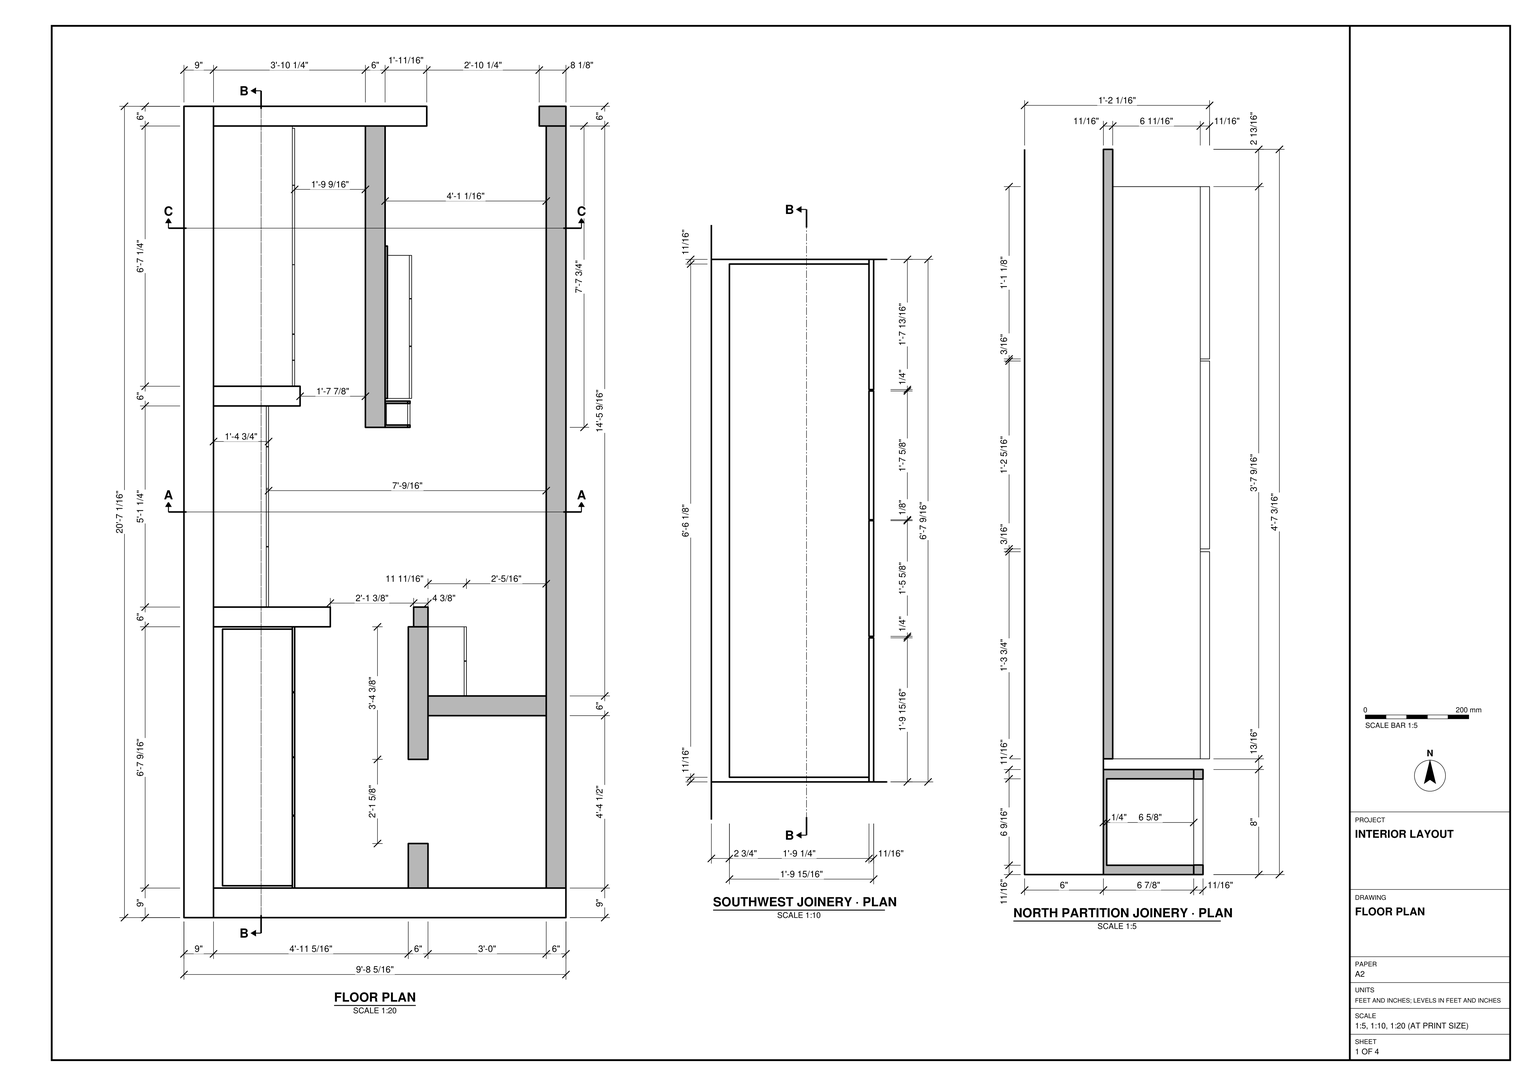
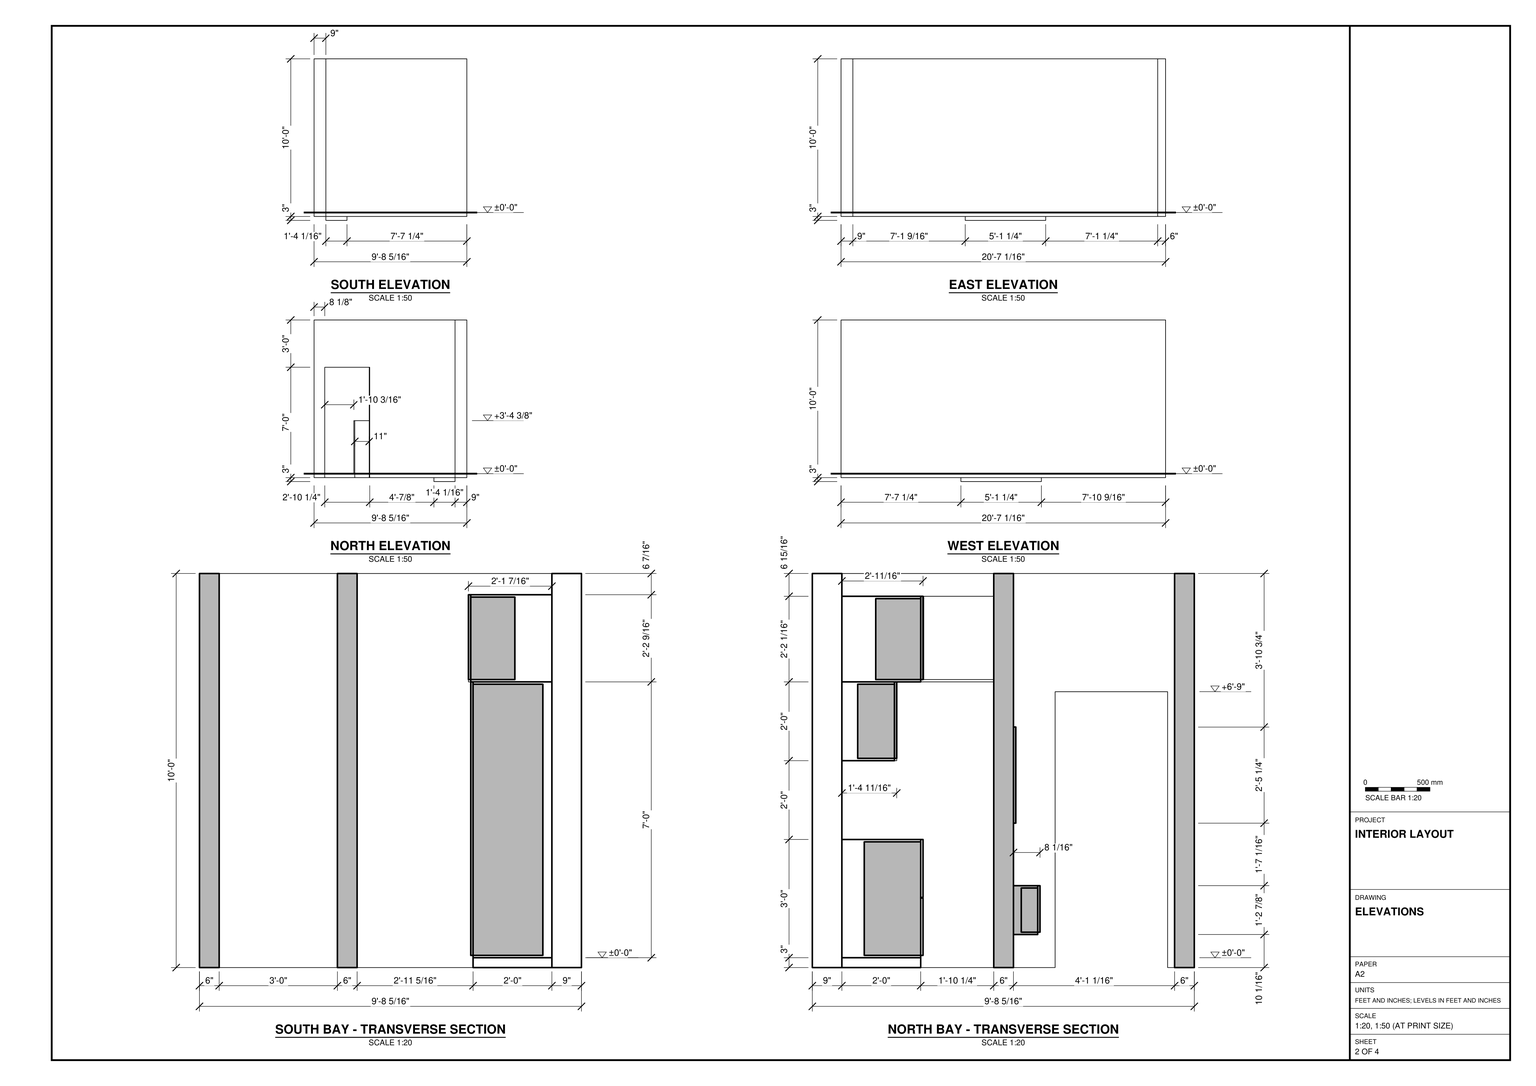
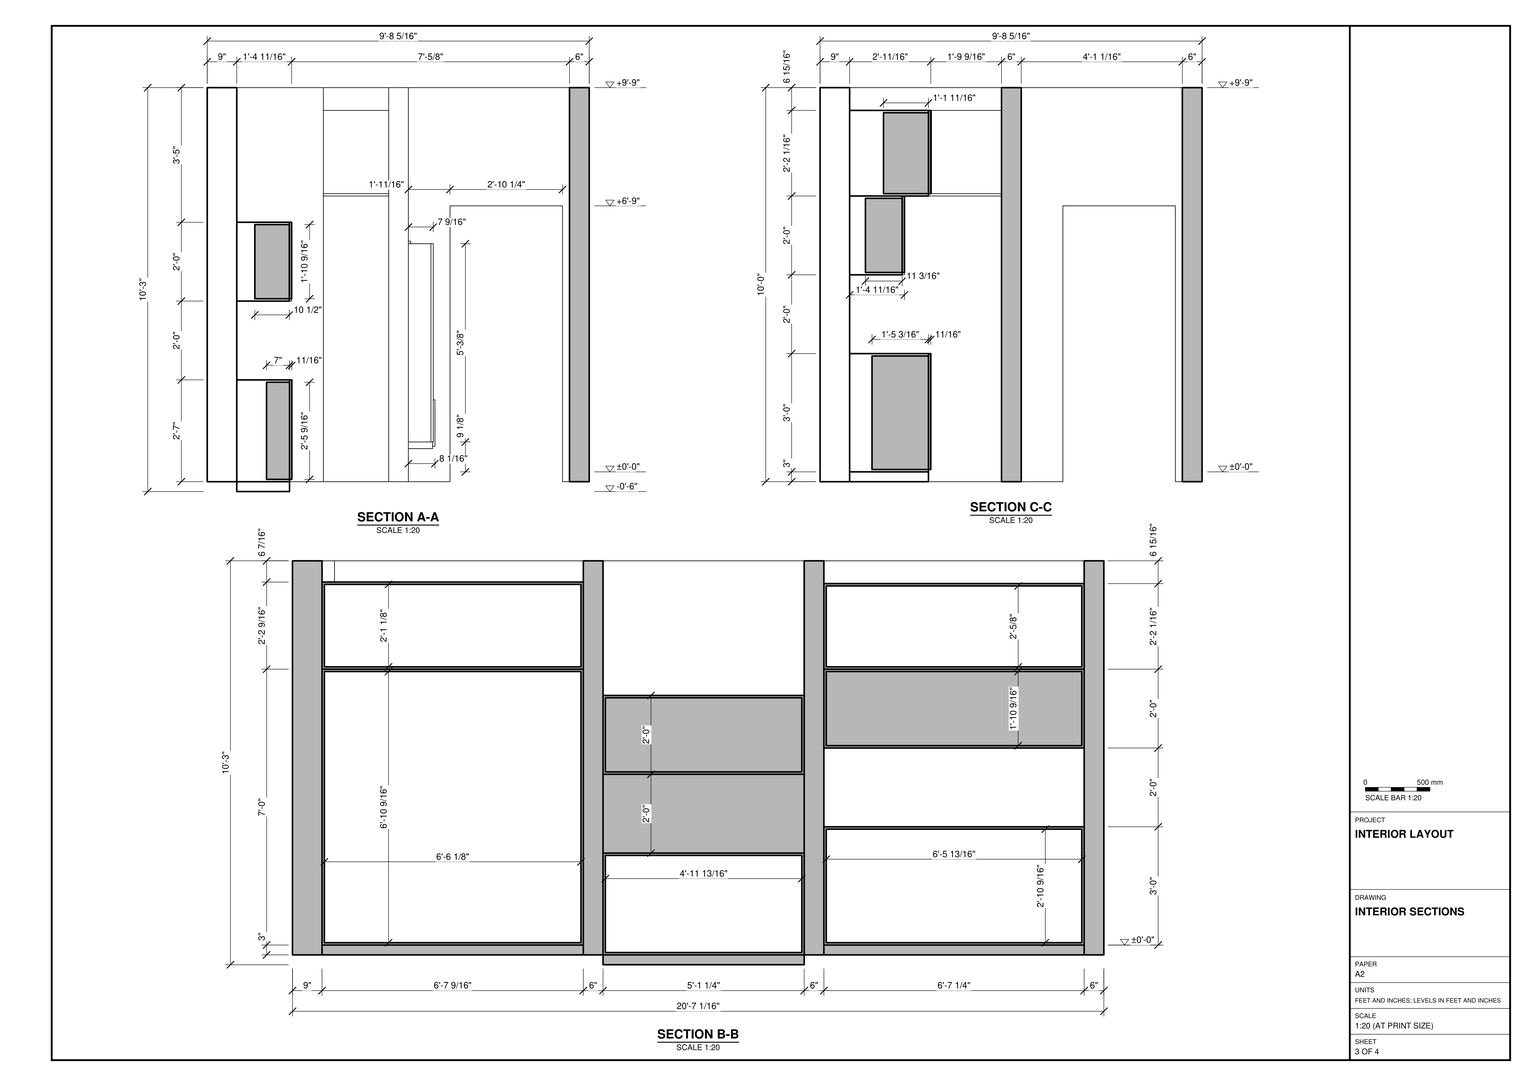
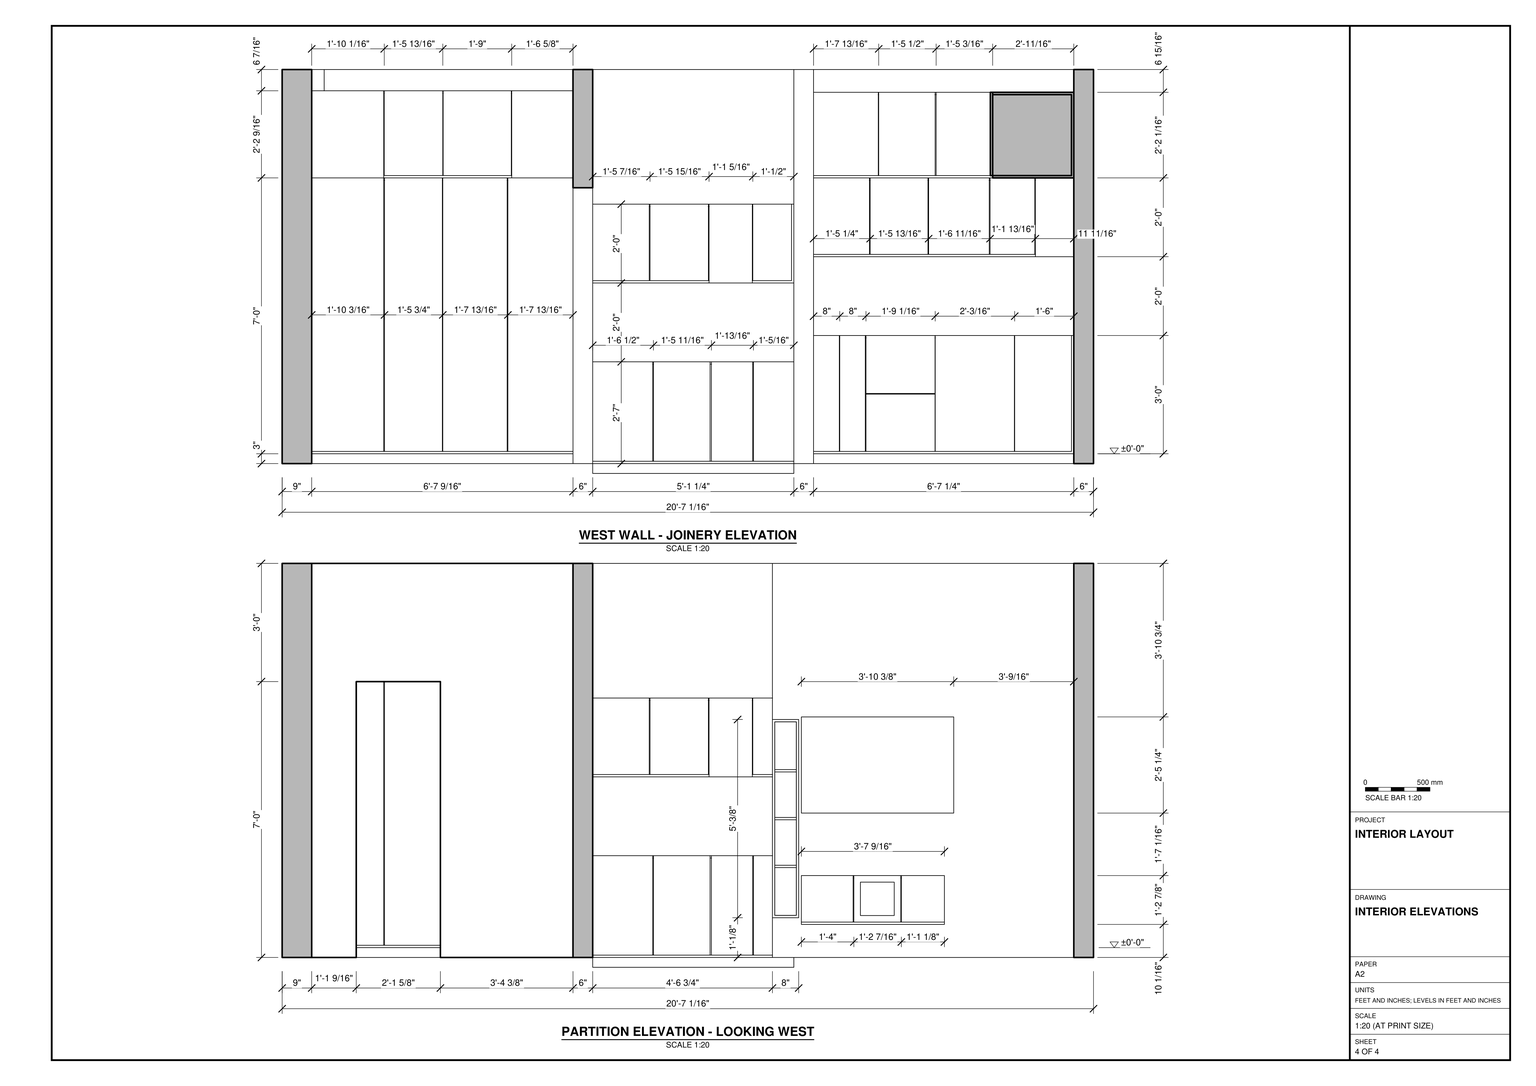
Build the interior shown in task_files/diagram_01.pdf in SketchUp. Work in feet and inches. The overall dimensions are 9'-8 5/16" east to west, 20'-7 1/16" north to south and 10'-3" high. Use ±0'-0" as the floor level for this single-storey layout.

Set out the 9" west and south walls, the 6" east and north walls, and the opening at the north end. Use the short returns from the west wall to divide the storage run into three bays. Follow the plan for the interrupted partition in the south bay, its connection to the east wall and the longer partition extending from the north wall.

Use section B-B to set the heights of the storage units. Fit the southwest bay with a tall cabinet and an overhead compartment. In the centre bay, leave a gap between the lower and upper units. In the northwest bay, model the base cabinet and both upper tiers, using the transverse section to set their different depths. Follow the detail plans for the cabinet fronts and the shallow units on the east face of the north partition.

Keep shell elements and each joinery or furniture piece in separate groups or components, and use components for repeated parts. Decor and loose items may be any suitable library components. Save one SketchUp model as output_files/three_bay_interior_with_built_in_storage.skp.

# SketchUp Ruby script. Lengths in inches.
U = 1.inch
M = Sketchup.active_model
def pt(a) = Geom::Point3d.new(a.map { |v| v * U })
def face(e, loops, mat)
  f = e.add_face(loops[0].map { |a| pt(a) })
  loops[1..].each { |l| e.add_face(l.map { |a| pt(a) }).erase! }
  f.material = f.back_material = mat if mat
  f
end
# faces: each face lists its corners as indices into pts; further lists are holes
def faces(e, pts, list, mat = nil) = list.each { |f| face(e, (f[0].is_a?(Array) ? f : [f]).map { |l| l.map { |i| pts[i] } }, mat) }
# xy, xz, yz: faces in a plane at the given z, y or x. An outline is a flat list of corners, or four numbers for a rectangle; further outlines are holes
def ring(l) = l.size == 4 ? [[l[0], l[1]], [l[2], l[1]], [l[2], l[3]], [l[0], l[3]]] : l.each_slice(2).to_a
def flat(e, list, mat, &to3) = list.each { |f| face(e, (f[0].is_a?(Array) ? f : [f]).map { |l| ring(l).map { |u, v| to3.(u, v) } }, mat) }
def xy(e, z, list, mat = nil) = flat(e, list, mat) { |x, y| [x, y, z] }
def xz(e, y, list, mat = nil) = flat(e, list, mat) { |x, z| [x, y, z] }
def yz(e, x, list, mat = nil) = flat(e, list, mat) { |y, z| [x, y, z] }
def lines(e, pts, list) = list.each { |a, b| e.add_line(pt(pts[a]), pt(pts[b])) }
# prism: a flat outline (further loops are holes) pulled along v
def prism(e, loops, v, mat = nil)
  f = face(e, loops, mat); d = Geom::Vector3d.new(v.map { |x| x * U })
  f.pushpull(f.normal.samedirection?(d) ? d.length : -d.length)
end
def box(e, o, s, mat = nil) = prism(e, [[o, [o[0] + s[0], o[1], o[2]], [o[0] + s[0], o[1] + s[1], o[2]], [o[0], o[1] + s[1], o[2]]]], [0, 0, s[2]], mat)
def at(x, y, z, deg = 0) = Geom::Transformation.translation(pt([x, y, z])) * Geom::Transformation.rotation(ORIGIN, Z_AXIS, deg.degrees)
def axes(o, x, y, z) = Geom::Transformation.new([*x, 0, *y, 0, *z, 0, *pt(o).to_a, 1])
def part(name) = M.definitions.add(name)
# library, detail: a bought-in or finely detailed component or shape, given as its bounding box
def library(name, o, s) = part(name).tap { |d| box(d.entities, o, s) }
def detail(e, o, s) = box(e.add_group.entities, o, s)
def put(e, d, t, mat = nil) = e.add_instance(d, t).tap { |i| i.material = mat if mat }
def group(e, t, mat = nil) = e.add_group.tap { |g| g.transformation = t; g.material = mat if mat }.entities
root = M.entities
c1 = part("Group\#56")
box(c1.entities,[0,0,0],[6.625,6.58,0.71])
xy(root,3.71,[[33,198.86,33.71,222.97]])
xy(root,39,[[33,198.86,33.71,222.97]])
xz(root,198.86,[[33,3.71,33.71,39]])
xz(root,222.97,[[33,3.71,33.71,39]])
yz(root,33,[[198.86,3.71,222.97,39]])
g1 = group(root,at(0,0,0))
prism(g1,[[[0,247.0625,0],[9,247.0625,0],[9,12.8,0],[9,0,0],[0,0,0]]],[0,0,120])
g2 = group(root,at(9,0,0))
box(g2,[0,0,0],[107.3125,9,120])
g3 = group(root,at(9,88.5625,0))
prism(g3,[[[0,0,0],[35.5625,0,0],[35.5625,0,84],[60.9375,0,84],[60.9375,0,0],[65.3125,0,0],[65.3125,0,120],[0,0,120]]],[0,6,0])
g4 = group(root,at(68.3125,9,0))
prism(g4,[[[6,0,0],[6,13.5625,0],[6,13.5625,84],[6,39.1875,84],[6,39.1875,0],[6,79.5625,0],[6,79.5625,120],[6,0,120]]],[-6,0,0])
g5 = group(root,at(110.3125,9,0))
box(g5,[0,0,0],[6,232.0625,120])
g6 = group(root,at(74.3125,61.5,0))
box(g6,[0,0,0],[36,6,120])
g7 = group(root,at(9,241.0625,0))
prism(g7,[[[99.1875,0,0],[107.3125,0,0],[107.3125,0,120],[0,0,120],[0,0,0],[64.9375,0,0],[64.9375,0,84],[99.1875,0,84]]],[0,6,0])
g8 = group(root,at(55.25,149.29,0))
box(g8,[0,0,0],[6,91.77,120])
g9 = group(root,at(9,155.8125,0))
box(g9,[0,0,0],[26.36,6,120])
g10 = group(root,at(9,161.8125,0))
box(g10,[0,0,0],[24,79.25,3])
g11 = group(root,at(9,161.8125,3))
xy(g11,0,[[0,0,24,79.25]])
xy(g11,0.71,[[6.8125,0.71,24,78.54]])
xy(g11,35.29,[[6.8125,0.71,24,78.54]])
xy(g11,36,[[0,0,24,79.25]])
xz(g11,0,[[0,0,24,36]])
xz(g11,0.71,[[6.8125,0.71,24,35.29]])
xz(g11,78.54,[[6.8125,0.71,24,35.29]])
xz(g11,79.25,[[0,0,24,36]])
yz(g11,0,[[0,0,79.25,36]])
yz(g11,6.8125,[[0.71,0.71,78.54,35.29]])
yz(g11,24,[[[0,0,79.25,36],[0.71,0.71,78.54,35.29]]])
g12 = group(root,at(33,161.8125,3.71))
box(g12,[0,0,0],[0.71,7.85,35.29])
g13 = group(root,at(33,169.79,3.71))
box(g13,[0,0,0],[0.71,7.77,35.29])
g14 = group(root,at(33,177.78,3.71))
xy(g14,0,[[0,0,0.71,21.02]])
xy(g14,17.45,[[0,0,0.71,21.02]])
xy(g14,17.65,[[0,0,0.71,21.02]])
xy(g14,35.29,[[0,0,0.71,21.02]])
xz(g14,0,[[0,0,0.71,17.45],[0,17.65,0.71,35.29]])
xz(g14,21.02,[[0,0,0.71,17.45],[0,17.65,0.71,35.29]])
yz(g14,0,[[0,0,21.02,17.45],[0,17.45,21.02,17.65],[0,17.65,21.02,35.29]])
yz(g14,0.71,[[0,0,21.02,17.45],[0,17.65,21.02,35.29]])
g15 = group(root,at(33.71,198.86,3.71))
yz(g15,0,[[0,0,24.1,35.29]])
g16 = group(root,at(33,223.0625,3.71))
box(g16,[0,0,0],[0.71,17.29,35.29])
g17 = group(root,at(9,161.8125,63))
xy(g17,0,[[0,0,16,79.25]])
xy(g17,0.71,[[4.8125,0.71,16,78.54]])
xy(g17,23.29,[[4.8125,0.71,16,78.54]])
xy(g17,24,[[0,0,16,79.25]])
xz(g17,0,[[0,0,16,24]])
xz(g17,0.71,[[4.8125,0.71,16,23.29]])
xz(g17,78.54,[[4.8125,0.71,16,23.29]])
xz(g17,79.25,[[0,0,16,24]])
yz(g17,0,[[0,0,79.25,24]])
yz(g17,4.8125,[[0.71,0.71,78.54,23.29]])
yz(g17,16,[[[0,0,79.25,24],[0.71,0.71,78.54,23.29]]])
g18 = group(root,at(25,161.8125,63.71))
box(g18,[0,0,0],[0.71,17.03,23.29])
g19 = group(root,at(25,179.05,63.71))
box(g19,[0,0,0],[0.71,17.6,23.29])
g20 = group(root,at(25,196.86,63.71))
box(g20,[0,0,0],[0.71,18.46,23.29])
g21 = group(root,at(25,215.5625,63.71))
box(g21,[0,0,0],[0.71,13.63,23.29])
g22 = group(root,at(25,229.35,63))
box(g22,[0,0,0],[0.71,11.71,24])
g23 = group(root,at(9,161.8125,87))
xy(g23,0,[[0,0,0,79.25,46.25,79.25,46.25,54.54,24,54.54,24,0]])
xy(g23,0.71,[[10.3125,0.71,24,0.71,24,54.54,46.25,54.54,46.25,78.54,10.3125,78.54]])
xy(g23,25.35,[[10.3125,0.71,10.3125,78.54,46.25,78.54,46.25,54.54,24,54.54,24,0.71]])
xy(g23,26.0625,[[0,0,24,0,24,54.54,46.25,54.54,46.25,79.25,0,79.25]])
xz(g23,0,[[0,0,24,26.0625]])
xz(g23,0.71,[[10.3125,0.71,24,25.35]])
xz(g23,54.54,[[24,0,46.25,0.71],[24,25.35,46.25,26.0625]])
xz(g23,78.54,[[10.3125,0.71,46.25,25.35]])
xz(g23,79.25,[[0,0,46.25,26.0625]])
yz(g23,0,[[0,0,79.25,26.0625]])
yz(g23,10.3125,[[0.71,0.71,78.54,25.35]])
yz(g23,24,[[0,0,54.54,0,54.54,0.71,0.71,0.71,0.71,25.35,54.54,25.35,54.54,26.0625,0,26.0625]])
yz(g23,46.25,[[54.54,0,79.25,0,79.25,26.0625,54.54,26.0625,54.54,25.35,78.54,25.35,78.54,0.71,54.54,0.71]])
g24 = group(root,at(33,161.8125,87.71))
box(g24,[0,0,0],[0.71,19.71,25.35])
g25 = group(root,at(33,181.65,87.71))
box(g25,[0,0,0],[0.71,17.18,25.35])
g26 = group(root,at(33,199.15,87.71))
box(g26,[0,0,0],[0.71,17.21,25.35])
g27 = group(root,at(33.95,215.65,87.71))
box(g27,[0,0,0],[21.3,0.71,25.35])
g28 = group(root,at(9,9,0))
box(g28,[0,0,0],[24,79.5625,3])
g29 = group(root,at(9,9,3))
xy(g29,0,[[0,0,24,79.5625]])
xy(g29,0.71,[[2.75,0.71,24,78.85]])
xy(g29,83.29,[[2.75,0.71,24,78.85]])
xy(g29,84,[[0,0,24,79.5625]])
xz(g29,0,[[0,0,24,84]])
xz(g29,0.71,[[2.75,0.71,24,83.29]])
xz(g29,78.85,[[2.75,0.71,24,83.29]])
xz(g29,79.5625,[[0,0,24,84]])
yz(g29,0,[[0,0,79.5625,84]])
yz(g29,2.75,[[0.71,0.71,78.85,83.29]])
yz(g29,24,[[[0,0,79.5625,84],[0.71,0.71,78.85,83.29]]])
g30 = group(root,at(33,9,3.71))
box(g30,[0,0,0],[0.71,21.93,83.29])
g31 = group(root,at(33,31.17,3.71))
box(g31,[0,0,0],[0.71,17.62,83.29])
g32 = group(root,at(33,48.92,3.71))
box(g32,[0,0,0],[0.71,19.6,83.29])
g33 = group(root,at(33,68.74,3.71))
box(g33,[0,0,0],[0.71,19.82,83.29])
g34 = group(root,at(9,9,87))
xy(g34,0,[[0,0,24.71,79.5625]])
xy(g34,0.71,[[11.27,0.71,24.71,78.85]])
xy(g34,25.83,[[11.27,0.71,24.71,78.85]])
xy(g34,26.54,[[0,0,24.71,79.5625]])
xz(g34,0,[[0,0,24.71,26.54]])
xz(g34,0.71,[[11.27,0.71,24.71,25.83]])
xz(g34,78.85,[[11.27,0.71,24.71,25.83]])
xz(g34,79.5625,[[0,0,24.71,26.54]])
yz(g34,0,[[0,0,79.5625,26.54]])
yz(g34,11.27,[[0.71,0.71,78.85,25.83]])
yz(g34,24.71,[[[0,0,79.5625,26.54],[0.71,0.71,78.85,25.83]]])
g35 = group(root,at(33.71,9,87))
box(g35,[0,0,0],[0.71,21.93,26.54])
g36 = group(root,at(33.71,31.08,87.71))
box(g36,[0,0,0],[0.71,17.83,25.83])
g37 = group(root,at(33.71,49.03,87.71))
box(g37,[0,0,0],[0.71,20.75,25.83])
g38 = group(root,at(33.71,69.91,87))
box(g38,[0,0,0],[0.71,18.65,26.54])
g39 = group(root,at(9,94.5625,0))
box(g39,[0,0,-3],[16.0625,61.25,3])
g40 = group(root,at(9,94.5625,0))
xy(g40,0,[[0,0,16.0625,61.25]])
xy(g40,0.71,[[9.0625,0.71,16.0625,60.54]])
xy(g40,30.29,[[9.0625,0.71,16.0625,60.54]])
xy(g40,31,[[0,0,16.0625,61.25]])
xz(g40,0,[[0,0,16.0625,31]])
xz(g40,0.71,[[9.0625,0.71,16.0625,30.29]])
xz(g40,60.54,[[9.0625,0.71,16.0625,30.29]])
xz(g40,61.25,[[0,0,16.0625,31]])
yz(g40,0,[[0,0,61.25,31]])
yz(g40,9.0625,[[0.71,0.71,60.54,30.29]])
yz(g40,16.0625,[[[0,0,61.25,31],[0.71,0.71,60.54,30.29]]])
g41 = group(root,at(25.0625,94.5625,0.71))
box(g41,[0,0,0],[0.71,18.3,30.29])
g42 = group(root,at(25.0625,113.05,0.71))
box(g42,[0,0,0],[0.71,17.25,30.29])
g43 = group(root,at(25.0625,130.71,0.71))
box(g43,[0,0,0],[0.71,12.59,30.29])
g44 = group(root,at(25.0625,143.5,0))
box(g44,[0,0,0.71],[0.71,12.3125,30.29])
g45 = group(root,at(9,94.5625,55))
xy(g45,0,[[0,0,16,61.25]])
xy(g45,0.71,[[5.5,0.71,16,60.54]])
xy(g45,23.29,[[5.5,0.71,16,60.54]])
xy(g45,24,[[0,0,16,61.25]])
xz(g45,0,[[0,0,16,24]])
xz(g45,0.71,[[5.5,0.71,16,23.29]])
xz(g45,60.54,[[5.5,0.71,16,23.29]])
xz(g45,61.25,[[0,0,16,24]])
yz(g45,0,[[0,0,61.25,24]])
yz(g45,5.5,[[0.71,0.71,60.54,23.29]])
yz(g45,16,[[[0,0,61.25,24],[0.71,0.71,60.54,23.29]]])
g46 = group(root,at(25,94.5625,55.71))
box(g46,[0,0,0],[0.71,17.21,23.29])
g47 = group(root,at(25,112.02,55.71))
box(g47,[0,0,0],[0.71,17.78,23.29])
g48 = group(root,at(25,129.99,55))
box(g48,[0,0,0],[0.71,13.18,24])
g49 = group(root,at(25,143.32,55.71))
box(g49,[0,0,0],[0.71,11.79,23.29])
g50 = group(root,at(61.25,158.1,10.0625))
xy(g50,0,[[0,0,7.375,43.5625]])
xy(g50,0.71,[[2.375,0.71,7.375,42.85]])
xy(g50,14.17,[[2.375,0.71,7.375,42.85]])
xy(g50,14.875,[[0,0,7.375,43.5625]])
xz(g50,0,[[0,0,7.375,14.875]])
xz(g50,0.71,[[2.375,0.71,7.375,14.17]])
xz(g50,42.85,[[2.375,0.71,7.375,14.17]])
xz(g50,43.5625,[[0,0,7.375,14.875]])
yz(g50,0,[[0,0,43.5625,14.875]])
yz(g50,2.375,[[0.71,0.71,42.85,14.17]])
yz(g50,7.375,[[[0,0,43.5625,14.875],[0.71,0.71,42.85,14.17]]])
g51 = group(root,at(68.625,158.1,10.77))
box(g51,[0,0,0],[0.71,15.77,14.17])
g52 = group(root,at(68.625,174.08,10.77))
prism(g52,[[[0.71,0,14.17],[0.71,0,0],[0.71,14.3,0],[0.71,14.3,14.17]],[[0.71,2,2],[0.71,2,12.17],[0.71,12.3,12.17],[0.71,12.3,2]]],[-0.71,0,0])
g53 = group(root,at(68.625,188.54,10.77))
box(g53,[0,0,0],[0.71,13.12,14.17])
g54 = group(root,at(61.25,158.1,43.97))
box(g54,[0,0,0],[0.71,46.4,29.28])
g55 = group(root,at(61.25,149.29,12.1))
xy(g55,0,[[0,0,6.875,8]])
xy(g55,0.71,[[0.25,0.71,6.875,7.29]])
xy(g55,59.67,[[0.25,0.71,6.875,7.29]])
xy(g55,60.375,[[0,0,6.875,8]])
xz(g55,0,[[0,0,6.875,60.375]])
xz(g55,0.71,[[0.25,0.71,6.875,59.67]])
xz(g55,7.29,[[0.25,0.71,6.875,59.67]])
xz(g55,8,[[0,0,6.875,60.375]])
yz(g55,0,[[0,0,8,60.375]])
yz(g55,0.25,[[0.71,0.71,7.29,59.67]])
yz(g55,6.875,[[[0,0,8,60.375],[0.71,0.71,7.29,59.67]]])
put(root,c1,at(61.5,150,27.37))
put(root,c1,at(61.5,150,41.93))
put(root,c1,at(61.5,150,56.49))
g56 = group(root,at(68.125,149.29,12.1))
prism(g56,[[[0.71,0,0],[0.71,8,0],[0.71,8,60.375],[0.71,0,60.375]],[[0.71,7.27,59.65],[0.71,7.27,0.73],[0.71,0.73,0.73],[0.71,0.73,59.65]]],[-0.71,0,0])
g57 = group(root,at(74.3125,67.5,0))
box(g57,[0,0,0],[11,21.0625,3])
g58 = group(root,at(74.3125,67.5,3))
xy(g58,0,[[0,0,11,21.0625]])
xy(g58,0.71,[[5.0625,0.71,11,20.35]])
xy(g58,39.67,[[5.0625,0.71,11,20.35]])
xy(g58,40.375,[[0,0,11,21.0625]])
xz(g58,0,[[0,0,11,40.375]])
xz(g58,0.71,[[5.0625,0.71,11,39.67]])
xz(g58,20.35,[[5.0625,0.71,11,39.67]])
xz(g58,21.0625,[[0,0,11,40.375]])
yz(g58,0,[[0,0,21.0625,40.375]])
yz(g58,5.0625,[[0.71,0.71,20.35,39.67]])
yz(g58,11,[[[0,0,21.0625,40.375],[0.71,0.71,20.35,39.67]]])
g59 = group(root,at(85.3125,67.5,3.71))
box(g59,[0,0,0],[0.71,10.53,39.67])
g60 = group(root,at(85.3125,78.21,3))
box(g60,[0,0,0],[0.71,10.35,40.375])
